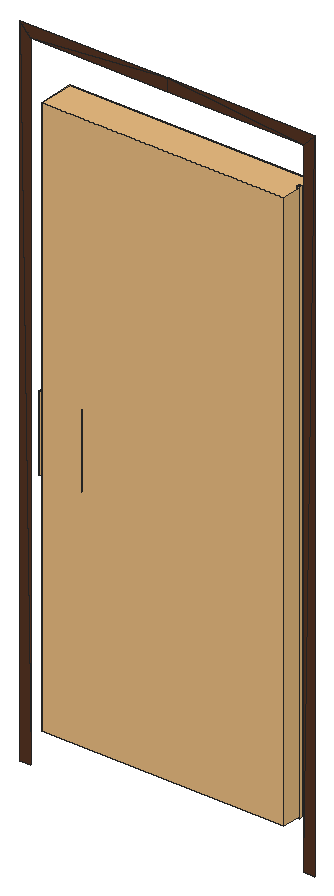
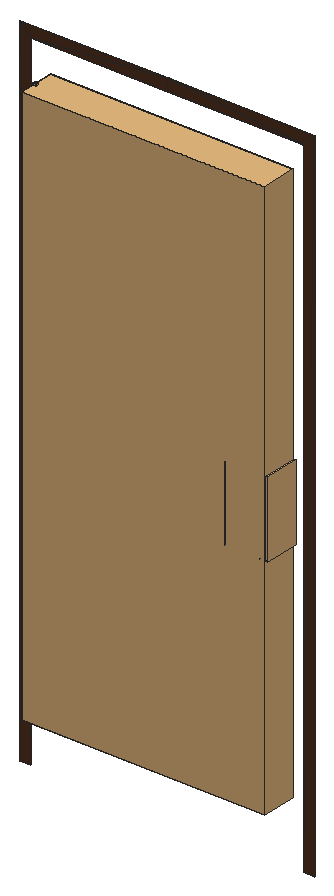
# SketchUp Ruby script. Lengths in inches.
U = 1.inch
M = Sketchup.active_model
def pt(a) = Geom::Point3d.new(a.map { |v| v * U })
def face(e, loops, mat)
  f = e.add_face(loops[0].map { |a| pt(a) })
  loops[1..].each { |l| e.add_face(l.map { |a| pt(a) }).erase! }
  f.material = f.back_material = mat if mat
  f
end
# faces: each face lists its corners as indices into pts; further lists are holes
def faces(e, pts, list, mat = nil) = list.each { |f| face(e, (f[0].is_a?(Array) ? f : [f]).map { |l| l.map { |i| pts[i] } }, mat) }
# xy, xz, yz: faces in a plane at the given z, y or x. An outline is a flat list of corners, or four numbers for a rectangle; further outlines are holes
def ring(l) = l.size == 4 ? [[l[0], l[1]], [l[2], l[1]], [l[2], l[3]], [l[0], l[3]]] : l.each_slice(2).to_a
def flat(e, list, mat, &to3) = list.each { |f| face(e, (f[0].is_a?(Array) ? f : [f]).map { |l| ring(l).map { |u, v| to3.(u, v) } }, mat) }
def xy(e, z, list, mat = nil) = flat(e, list, mat) { |x, y| [x, y, z] }
def xz(e, y, list, mat = nil) = flat(e, list, mat) { |x, z| [x, y, z] }
def yz(e, x, list, mat = nil) = flat(e, list, mat) { |y, z| [x, y, z] }
def lines(e, pts, list) = list.each { |a, b| e.add_line(pt(pts[a]), pt(pts[b])) }
# prism: a flat outline (further loops are holes) pulled along v
def prism(e, loops, v, mat = nil)
  f = face(e, loops, mat); d = Geom::Vector3d.new(v.map { |x| x * U })
  f.pushpull(f.normal.samedirection?(d) ? d.length : -d.length)
end
def box(e, o, s, mat = nil) = prism(e, [[o, [o[0] + s[0], o[1], o[2]], [o[0] + s[0], o[1] + s[1], o[2]], [o[0], o[1] + s[1], o[2]]]], [0, 0, s[2]], mat)
def at(x, y, z, deg = 0) = Geom::Transformation.translation(pt([x, y, z])) * Geom::Transformation.rotation(ORIGIN, Z_AXIS, deg.degrees)
def axes(o, x, y, z) = Geom::Transformation.new([*x, 0, *y, 0, *z, 0, *pt(o).to_a, 1])
def part(name) = M.definitions.add(name)
# library, detail: a bought-in or finely detailed component or shape, given as its bounding box
def library(name, o, s) = part(name).tap { |d| box(d.entities, o, s) }
def detail(e, o, s) = box(e.add_group.entities, o, s)
def put(e, d, t, mat = nil) = e.add_instance(d, t).tap { |i| i.material = mat if mat }
def group(e, t, mat = nil) = e.add_group.tap { |g| g.transformation = t; g.material = mat if mat }.entities
root = M.entities
M.materials.add("Material \#0").color = [86, 53, 35]
M.materials.add("Material \#1").color = [140, 140, 140]
c1 = library("3DGeom~3_Defintion",[-83.33,-500,-350],[620.1,1000,533.33])
c2 = part("3DGeom~21_Defintion")
xy(c2.entities,73.08,[[-976.3,-241.71,23.7,-241.71,-976.3,-223.46],[23.7,-241.71,5.45,-223.46,-976.3,-223.46],[23.7,-241.71,23.7,0,5.45,-223.46],[5.45,-223.46,23.7,0,5.45,0],[23.7,0,23.7,241.71,5.45,223.46],
  [5.45,0,23.7,0,5.45,223.46],[-976.3,223.46,23.7,241.71,-976.3,241.71],[-976.3,223.46,5.45,223.46,23.7,241.71]],"Material \#0")
c3 = library("3DGeom~6_Defintion",[-5.59,-471.8,-48.03],[468.87,1000,73.72])
c4 = library("3DGeom~9_Defintion",[456.52,-471.89,-18.89],[5.57,1000,5.49])
c5 = library("3DGeom~7_Defintion",[455.56,-471.94,-18.85],[5.55,1000,5.48])
c6 = part("3DGeom~8_Defintion")
xz(c6.entities,-471.94,[[458.125,-17.29,459.53,-16.11,457.73,-17.15],[458.125,-17.29,458.54,-17.29,459.53,-16.11],[458.54,-17.29,458.93,-17.15,459.53,-16.11],[457.73,-17.15,459.53,-16.11,457.42,-16.88],[458.93,-17.15,459.25,-16.88,459.53,-16.11],
  [457.42,-16.88,459.53,-16.11,457.21,-16.52],[459.25,-16.88,459.46,-16.52,459.53,-16.11],[457.21,-16.52,459.53,-16.11,457.14,-16.11],[457.14,-16.11,459.53,-16.11,457.21,-15.7],[459.53,-16.11,457.42,-15.34,457.21,-15.7],
  [459.53,-16.11,457.73,-15.07,457.42,-15.34],[459.53,-16.11,458.125,-14.93,457.73,-15.07],[459.53,-16.11,458.54,-14.93,458.125,-14.93],[459.53,-16.11,458.93,-15.07,458.54,-14.93],[459.53,-16.11,459.25,-15.34,458.93,-15.07],
  [459.53,-16.11,459.46,-15.7,459.25,-15.34]],"Material \#1")
xz(c6.entities,-416.39,[[458.125,-17.29,457.73,-17.15,459.53,-16.11],[458.125,-17.29,459.53,-16.11,458.54,-17.29],[458.54,-17.29,459.53,-16.11,458.93,-17.15],[457.73,-17.15,457.42,-16.88,459.53,-16.11],[458.93,-17.15,459.53,-16.11,459.25,-16.88],
  [457.42,-16.88,457.21,-16.52,459.53,-16.11],[459.25,-16.88,459.53,-16.11,459.46,-16.52],[457.21,-16.52,457.14,-16.11,459.53,-16.11],[457.14,-16.11,457.21,-15.7,459.53,-16.11],[459.53,-16.11,457.21,-15.7,457.42,-15.34],
  [459.53,-16.11,457.42,-15.34,457.73,-15.07],[459.53,-16.11,457.73,-15.07,458.125,-14.93],[459.53,-16.11,458.125,-14.93,458.54,-14.93],[459.53,-16.11,458.54,-14.93,458.93,-15.07],[459.53,-16.11,458.93,-15.07,459.25,-15.34],
  [459.53,-16.11,459.25,-15.34,459.46,-15.7]],"Material \#1")
xz(c6.entities,-27.5,[[458.125,-17.29,459.53,-16.11,457.73,-17.15],[458.125,-17.29,458.54,-17.29,459.53,-16.11],[458.54,-17.29,458.93,-17.15,459.53,-16.11],[457.73,-17.15,459.53,-16.11,457.42,-16.88],[458.93,-17.15,459.25,-16.88,459.53,-16.11],
  [457.42,-16.88,459.53,-16.11,457.21,-16.52],[459.25,-16.88,459.46,-16.52,459.53,-16.11],[457.21,-16.52,459.53,-16.11,457.14,-16.11],[457.14,-16.11,459.53,-16.11,457.21,-15.7],[459.53,-16.11,457.42,-15.34,457.21,-15.7],
  [459.53,-16.11,457.73,-15.07,457.42,-15.34],[459.53,-16.11,458.125,-14.93,457.73,-15.07],[459.53,-16.11,458.54,-14.93,458.125,-14.93],[459.53,-16.11,458.93,-15.07,458.54,-14.93],[459.53,-16.11,459.25,-15.34,458.93,-15.07],
  [459.53,-16.11,459.46,-15.7,459.25,-15.34]],"Material \#1")
xz(c6.entities,28.06,[[458.125,-17.29,457.73,-17.15,459.53,-16.11],[458.125,-17.29,459.53,-16.11,458.54,-17.29],[458.54,-17.29,459.53,-16.11,458.93,-17.15],[457.73,-17.15,457.42,-16.88,459.53,-16.11],[458.93,-17.15,459.53,-16.11,459.25,-16.88],
  [457.42,-16.88,457.21,-16.52,459.53,-16.11],[459.25,-16.88,459.53,-16.11,459.46,-16.52],[457.21,-16.52,457.14,-16.11,459.53,-16.11],[457.14,-16.11,457.21,-15.7,459.53,-16.11],[459.53,-16.11,457.21,-15.7,457.42,-15.34],
  [459.53,-16.11,457.42,-15.34,457.73,-15.07],[459.53,-16.11,457.73,-15.07,458.125,-14.93],[459.53,-16.11,458.125,-14.93,458.54,-14.93],[459.53,-16.11,458.54,-14.93,458.93,-15.07],[459.53,-16.11,458.93,-15.07,459.25,-15.34],
  [459.53,-16.11,459.25,-15.34,459.46,-15.7]],"Material \#1")
xz(c6.entities,472.5,[[458.125,-17.29,459.53,-16.11,457.73,-17.15],[458.125,-17.29,458.54,-17.29,459.53,-16.11],[458.54,-17.29,458.93,-17.15,459.53,-16.11],[457.73,-17.15,459.53,-16.11,457.42,-16.88],[458.93,-17.15,459.25,-16.88,459.53,-16.11],
  [457.42,-16.88,459.53,-16.11,457.21,-16.52],[459.25,-16.88,459.46,-16.52,459.53,-16.11],[457.21,-16.52,459.53,-16.11,457.14,-16.11],[457.14,-16.11,459.53,-16.11,457.21,-15.7],[459.53,-16.11,457.42,-15.34,457.21,-15.7],
  [459.53,-16.11,457.73,-15.07,457.42,-15.34],[459.53,-16.11,458.125,-14.93,457.73,-15.07],[459.53,-16.11,458.54,-14.93,458.125,-14.93],[459.53,-16.11,458.93,-15.07,458.54,-14.93],[459.53,-16.11,459.25,-15.34,458.93,-15.07],
  [459.53,-16.11,459.46,-15.7,459.25,-15.34]],"Material \#1")
xz(c6.entities,528.06,[[458.125,-17.29,457.73,-17.15,459.53,-16.11],[458.125,-17.29,459.53,-16.11,458.54,-17.29],[458.54,-17.29,459.53,-16.11,458.93,-17.15],[457.73,-17.15,457.42,-16.88,459.53,-16.11],[458.93,-17.15,459.53,-16.11,459.25,-16.88],
  [457.42,-16.88,457.21,-16.52,459.53,-16.11],[459.25,-16.88,459.53,-16.11,459.46,-16.52],[457.21,-16.52,457.14,-16.11,459.53,-16.11],[457.14,-16.11,457.21,-15.7,459.53,-16.11],[459.53,-16.11,457.21,-15.7,457.42,-15.34],
  [459.53,-16.11,457.42,-15.34,457.73,-15.07],[459.53,-16.11,457.73,-15.07,458.125,-14.93],[459.53,-16.11,458.125,-14.93,458.54,-14.93],[459.53,-16.11,458.54,-14.93,458.93,-15.07],[459.53,-16.11,458.93,-15.07,459.25,-15.34],
  [459.53,-16.11,459.25,-15.34,459.46,-15.7]],"Material \#1")
xy(root,9.094,[[138.948,197.844,138.952,197.861,138.889,197.864],[138.948,197.844,139.008,197.861,138.952,197.861],[138.948,197.844,139.011,197.844,139.008,197.861],[139.011,197.844,139.061,197.878,139.008,197.861],[139.011,197.844,139.07,197.864,139.061,197.878],
  [138.952,197.861,138.898,197.878,138.889,197.864],[138.889,197.864,138.898,197.878,138.841,197.901],[139.07,197.864,139.104,197.912,139.061,197.878],[139.07,197.864,139.118,197.901,139.104,197.912],[138.898,197.878,138.855,197.912,138.841,197.901],
  [138.841,197.901,138.855,197.912,138.81,197.952],[139.118,197.901,139.132,197.958,139.104,197.912],[139.118,197.901,139.149,197.952,139.132,197.958],[138.855,197.912,138.827,197.958,138.81,197.952],[138.81,197.952,138.827,197.958,138.799,198.009],
  [139.149,197.952,139.142,198.009,139.132,197.958],[139.149,197.952,139.16,198.009,139.142,198.009],[138.827,197.958,138.817,198.009,138.799,198.009],[138.799,198.009,138.817,198.009,138.81,198.067],[138.817,198.009,138.827,198.061,138.81,198.067],
  [139.142,198.009,139.16,198.009,139.132,198.061],[139.16,198.009,139.149,198.067,139.132,198.061],[138.827,198.061,138.841,198.117,138.81,198.067],[138.827,198.061,138.855,198.106,138.841,198.117],[139.132,198.061,139.149,198.067,139.104,198.106],
  [139.149,198.067,139.118,198.117,139.104,198.106],[138.855,198.106,138.889,198.155,138.841,198.117],[138.855,198.106,138.898,198.14,138.889,198.155],[139.104,198.106,139.118,198.117,139.061,198.14],[139.118,198.117,139.07,198.155,139.061,198.14],
  [138.898,198.14,138.948,198.175,138.889,198.155],[138.898,198.14,138.952,198.158,138.948,198.175],[139.061,198.14,139.07,198.155,139.008,198.158],[139.07,198.155,139.011,198.175,139.008,198.158],[138.952,198.158,139.011,198.175,138.948,198.175],
  [138.952,198.158,139.008,198.158,139.011,198.175]],"Material \#1")
xy(root,9.11,[[138.948,197.844,138.889,197.864,138.898,197.878],[138.948,197.844,138.898,197.878,138.952,197.861],[138.948,197.844,138.952,197.861,139.011,197.844],[139.011,197.844,138.952,197.861,139.008,197.861],[139.011,197.844,139.008,197.861,139.07,197.864],
  [139.008,197.861,139.061,197.878,139.07,197.864],[138.889,197.864,138.841,197.901,138.855,197.912],[138.889,197.864,138.855,197.912,138.898,197.878],[139.07,197.864,139.061,197.878,139.118,197.901],[139.061,197.878,139.104,197.912,139.118,197.901],
  [138.841,197.901,138.81,197.952,138.827,197.958],[138.841,197.901,138.827,197.958,138.855,197.912],[139.118,197.901,139.104,197.912,139.149,197.952],[139.104,197.912,139.132,197.958,139.149,197.952],[138.81,197.952,138.799,198.009,138.817,198.009],
  [138.81,197.952,138.817,198.009,138.827,197.958],[139.149,197.952,139.132,197.958,139.16,198.009],[139.132,197.958,139.142,198.009,139.16,198.009],[138.799,198.009,138.81,198.067,138.827,198.061],[138.799,198.009,138.827,198.061,138.817,198.009],
  [139.142,198.009,139.132,198.061,139.149,198.067],[139.142,198.009,139.149,198.067,139.16,198.009],[138.827,198.061,138.81,198.067,138.855,198.106],[139.132,198.061,139.104,198.106,139.118,198.117],[139.132,198.061,139.118,198.117,139.149,198.067],
  [138.81,198.067,138.841,198.117,138.855,198.106],[138.855,198.106,138.841,198.117,138.898,198.14],[139.104,198.106,139.061,198.14,139.07,198.155],[139.104,198.106,139.07,198.155,139.118,198.117],[138.841,198.117,138.889,198.155,138.898,198.14],
  [138.898,198.14,138.889,198.155,138.952,198.158],[139.061,198.14,139.008,198.158,139.011,198.175],[139.061,198.14,139.011,198.175,139.07,198.155],[138.889,198.155,138.948,198.175,138.952,198.158],[138.952,198.158,138.948,198.175,139.008,198.158],
  [139.008,198.158,138.948,198.175,139.011,198.175]],"Material \#1")
xy(root,12.631,[[138.948,197.844,138.898,197.878,138.889,197.864],[138.948,197.844,138.952,197.861,138.898,197.878],[138.948,197.844,139.011,197.844,138.952,197.861],[139.011,197.844,139.008,197.861,138.952,197.861],[139.011,197.844,139.07,197.864,139.008,197.861],
  [139.008,197.861,139.07,197.864,139.061,197.878],[138.889,197.864,138.855,197.912,138.841,197.901],[138.889,197.864,138.898,197.878,138.855,197.912],[139.07,197.864,139.118,197.901,139.061,197.878],[139.061,197.878,139.118,197.901,139.104,197.912],
  [138.841,197.901,138.827,197.958,138.81,197.952],[138.841,197.901,138.855,197.912,138.827,197.958],[139.118,197.901,139.149,197.952,139.104,197.912],[139.104,197.912,139.149,197.952,139.132,197.958],[138.81,197.952,138.817,198.009,138.799,198.009],
  [138.81,197.952,138.827,197.958,138.817,198.009],[139.149,197.952,139.16,198.009,139.132,197.958],[139.132,197.958,139.16,198.009,139.142,198.009],[138.799,198.009,138.817,198.009,138.827,198.061],[138.799,198.009,138.827,198.061,138.81,198.067],
  [139.142,198.009,139.149,198.067,139.132,198.061],[139.142,198.009,139.16,198.009,139.149,198.067],[138.827,198.061,138.855,198.106,138.81,198.067],[139.132,198.061,139.118,198.117,139.104,198.106],[139.132,198.061,139.149,198.067,139.118,198.117],
  [138.81,198.067,138.855,198.106,138.841,198.117],[138.855,198.106,138.898,198.14,138.841,198.117],[139.104,198.106,139.07,198.155,139.061,198.14],[139.104,198.106,139.118,198.117,139.07,198.155],[138.841,198.117,138.898,198.14,138.889,198.155],
  [138.898,198.14,138.952,198.158,138.889,198.155],[139.061,198.14,139.011,198.175,139.008,198.158],[139.061,198.14,139.07,198.155,139.011,198.175],[138.889,198.155,138.952,198.158,138.948,198.175],[138.952,198.158,139.008,198.158,138.948,198.175],
  [139.008,198.158,139.011,198.175,138.948,198.175]],"Material \#1")
xy(root,12.646,[[138.948,197.844,138.889,197.864,138.952,197.861],[138.948,197.844,138.952,197.861,139.008,197.861],[138.948,197.844,139.008,197.861,139.011,197.844],[139.011,197.844,139.008,197.861,139.061,197.878],[139.011,197.844,139.061,197.878,139.07,197.864],
  [138.952,197.861,138.889,197.864,138.898,197.878],[138.889,197.864,138.841,197.901,138.898,197.878],[139.07,197.864,139.061,197.878,139.104,197.912],[139.07,197.864,139.104,197.912,139.118,197.901],[138.898,197.878,138.841,197.901,138.855,197.912],
  [138.841,197.901,138.81,197.952,138.855,197.912],[139.118,197.901,139.104,197.912,139.132,197.958],[139.118,197.901,139.132,197.958,139.149,197.952],[138.855,197.912,138.81,197.952,138.827,197.958],[138.81,197.952,138.799,198.009,138.827,197.958],
  [139.149,197.952,139.132,197.958,139.142,198.009],[139.149,197.952,139.142,198.009,139.16,198.009],[138.827,197.958,138.799,198.009,138.817,198.009],[138.799,198.009,138.81,198.067,138.817,198.009],[138.817,198.009,138.81,198.067,138.827,198.061],
  [139.142,198.009,139.132,198.061,139.16,198.009],[139.16,198.009,139.132,198.061,139.149,198.067],[138.827,198.061,138.81,198.067,138.841,198.117],[138.827,198.061,138.841,198.117,138.855,198.106],[139.132,198.061,139.104,198.106,139.149,198.067],
  [139.149,198.067,139.104,198.106,139.118,198.117],[138.855,198.106,138.841,198.117,138.889,198.155],[138.855,198.106,138.889,198.155,138.898,198.14],[139.104,198.106,139.061,198.14,139.118,198.117],[139.118,198.117,139.061,198.14,139.07,198.155],
  [138.898,198.14,138.889,198.155,138.948,198.175],[138.898,198.14,138.948,198.175,138.952,198.158],[139.061,198.14,139.008,198.158,139.07,198.155],[139.07,198.155,139.008,198.158,139.011,198.175],[138.952,198.158,138.948,198.175,139.011,198.175],
  [138.952,198.158,139.011,198.175,139.008,198.158]],"Material \#1")
xy(root,40.496,[[138.948,197.844,138.952,197.861,138.889,197.864],[138.948,197.844,139.008,197.861,138.952,197.861],[138.948,197.844,139.011,197.844,139.008,197.861],[139.011,197.844,139.061,197.878,139.008,197.861],[139.011,197.844,139.07,197.864,139.061,197.878],
  [138.952,197.861,138.898,197.878,138.889,197.864],[138.889,197.864,138.898,197.878,138.841,197.901],[139.07,197.864,139.104,197.912,139.061,197.878],[139.07,197.864,139.118,197.901,139.104,197.912],[138.898,197.878,138.855,197.912,138.841,197.901],
  [138.841,197.901,138.855,197.912,138.81,197.952],[139.118,197.901,139.132,197.958,139.104,197.912],[139.118,197.901,139.149,197.952,139.132,197.958],[138.855,197.912,138.827,197.958,138.81,197.952],[138.81,197.952,138.827,197.958,138.799,198.009],
  [139.149,197.952,139.142,198.009,139.132,197.958],[139.149,197.952,139.16,198.009,139.142,198.009],[138.827,197.958,138.817,198.009,138.799,198.009],[138.799,198.009,138.817,198.009,138.81,198.067],[138.817,198.009,138.827,198.061,138.81,198.067],
  [139.142,198.009,139.16,198.009,139.132,198.061],[139.16,198.009,139.149,198.067,139.132,198.061],[138.827,198.061,138.841,198.117,138.81,198.067],[138.827,198.061,138.855,198.106,138.841,198.117],[139.132,198.061,139.149,198.067,139.104,198.106],
  [139.149,198.067,139.118,198.117,139.104,198.106],[138.855,198.106,138.889,198.155,138.841,198.117],[138.855,198.106,138.898,198.14,138.889,198.155],[139.104,198.106,139.118,198.117,139.061,198.14],[139.118,198.117,139.07,198.155,139.061,198.14],
  [138.898,198.14,138.948,198.175,138.889,198.155],[138.898,198.14,138.952,198.158,138.948,198.175],[139.061,198.14,139.07,198.155,139.008,198.158],[139.07,198.155,139.011,198.175,139.008,198.158],[138.952,198.158,139.011,198.175,138.948,198.175],
  [138.952,198.158,139.008,198.158,139.011,198.175]],"Material \#1")
xy(root,40.511,[[138.948,197.844,138.889,197.864,138.898,197.878],[138.948,197.844,138.898,197.878,138.952,197.861],[138.948,197.844,138.952,197.861,139.011,197.844],[139.011,197.844,138.952,197.861,139.008,197.861],[139.011,197.844,139.008,197.861,139.07,197.864],
  [139.008,197.861,139.061,197.878,139.07,197.864],[138.889,197.864,138.841,197.901,138.855,197.912],[138.889,197.864,138.855,197.912,138.898,197.878],[139.07,197.864,139.061,197.878,139.118,197.901],[139.061,197.878,139.104,197.912,139.118,197.901],
  [138.841,197.901,138.81,197.952,138.827,197.958],[138.841,197.901,138.827,197.958,138.855,197.912],[139.118,197.901,139.104,197.912,139.149,197.952],[139.104,197.912,139.132,197.958,139.149,197.952],[138.81,197.952,138.799,198.009,138.817,198.009],
  [138.81,197.952,138.817,198.009,138.827,197.958],[139.149,197.952,139.132,197.958,139.16,198.009],[139.132,197.958,139.142,198.009,139.16,198.009],[138.799,198.009,138.81,198.067,138.827,198.061],[138.799,198.009,138.827,198.061,138.817,198.009],
  [139.142,198.009,139.132,198.061,139.149,198.067],[139.142,198.009,139.149,198.067,139.16,198.009],[138.827,198.061,138.81,198.067,138.855,198.106],[139.132,198.061,139.104,198.106,139.118,198.117],[139.132,198.061,139.118,198.117,139.149,198.067],
  [138.81,198.067,138.841,198.117,138.855,198.106],[138.855,198.106,138.841,198.117,138.898,198.14],[139.104,198.106,139.061,198.14,139.07,198.155],[139.104,198.106,139.07,198.155,139.118,198.117],[138.841,198.117,138.889,198.155,138.898,198.14],
  [138.898,198.14,138.889,198.155,138.952,198.158],[139.061,198.14,139.008,198.158,139.011,198.175],[139.061,198.14,139.011,198.175,139.07,198.155],[138.889,198.155,138.948,198.175,138.952,198.158],[138.952,198.158,138.948,198.175,139.008,198.158],
  [139.008,198.158,138.948,198.175,139.011,198.175]],"Material \#1")
xy(root,44.032,[[138.948,197.844,138.898,197.878,138.889,197.864],[138.948,197.844,138.952,197.861,138.898,197.878],[138.948,197.844,139.011,197.844,138.952,197.861],[139.011,197.844,139.008,197.861,138.952,197.861],[139.011,197.844,139.07,197.864,139.008,197.861],
  [139.008,197.861,139.07,197.864,139.061,197.878],[138.889,197.864,138.855,197.912,138.841,197.901],[138.889,197.864,138.898,197.878,138.855,197.912],[139.07,197.864,139.118,197.901,139.061,197.878],[139.061,197.878,139.118,197.901,139.104,197.912],
  [138.841,197.901,138.827,197.958,138.81,197.952],[138.841,197.901,138.855,197.912,138.827,197.958],[139.118,197.901,139.149,197.952,139.104,197.912],[139.104,197.912,139.149,197.952,139.132,197.958],[138.81,197.952,138.817,198.009,138.799,198.009],
  [138.81,197.952,138.827,197.958,138.817,198.009],[139.149,197.952,139.16,198.009,139.132,197.958],[139.132,197.958,139.16,198.009,139.142,198.009],[138.799,198.009,138.817,198.009,138.827,198.061],[138.799,198.009,138.827,198.061,138.81,198.067],
  [139.142,198.009,139.149,198.067,139.132,198.061],[139.142,198.009,139.16,198.009,139.149,198.067],[138.827,198.061,138.855,198.106,138.81,198.067],[139.132,198.061,139.118,198.117,139.104,198.106],[139.132,198.061,139.149,198.067,139.118,198.117],
  [138.81,198.067,138.855,198.106,138.841,198.117],[138.855,198.106,138.898,198.14,138.841,198.117],[139.104,198.106,139.07,198.155,139.061,198.14],[139.104,198.106,139.118,198.117,139.07,198.155],[138.841,198.117,138.898,198.14,138.889,198.155],
  [138.898,198.14,138.952,198.158,138.889,198.155],[139.061,198.14,139.011,198.175,139.008,198.158],[139.061,198.14,139.07,198.155,139.011,198.175],[138.889,198.155,138.952,198.158,138.948,198.175],[138.952,198.158,139.008,198.158,138.948,198.175],
  [139.008,198.158,139.011,198.175,138.948,198.175]],"Material \#1")
xy(root,44.048,[[138.948,197.844,138.889,197.864,138.952,197.861],[138.948,197.844,138.952,197.861,139.008,197.861],[138.948,197.844,139.008,197.861,139.011,197.844],[139.011,197.844,139.008,197.861,139.061,197.878],[139.011,197.844,139.061,197.878,139.07,197.864],
  [138.952,197.861,138.889,197.864,138.898,197.878],[138.889,197.864,138.841,197.901,138.898,197.878],[139.07,197.864,139.061,197.878,139.104,197.912],[139.07,197.864,139.104,197.912,139.118,197.901],[138.898,197.878,138.841,197.901,138.855,197.912],
  [138.841,197.901,138.81,197.952,138.855,197.912],[139.118,197.901,139.104,197.912,139.132,197.958],[139.118,197.901,139.132,197.958,139.149,197.952],[138.855,197.912,138.81,197.952,138.827,197.958],[138.81,197.952,138.799,198.009,138.827,197.958],
  [139.149,197.952,139.132,197.958,139.142,198.009],[139.149,197.952,139.142,198.009,139.16,198.009],[138.827,197.958,138.799,198.009,138.817,198.009],[138.799,198.009,138.81,198.067,138.817,198.009],[138.817,198.009,138.81,198.067,138.827,198.061],
  [139.142,198.009,139.132,198.061,139.16,198.009],[139.16,198.009,139.132,198.061,139.149,198.067],[138.827,198.061,138.81,198.067,138.841,198.117],[138.827,198.061,138.841,198.117,138.855,198.106],[139.132,198.061,139.104,198.106,139.149,198.067],
  [139.149,198.067,139.104,198.106,139.118,198.117],[138.855,198.106,138.841,198.117,138.889,198.155],[138.855,198.106,138.889,198.155,138.898,198.14],[139.104,198.106,139.061,198.14,139.118,198.117],[139.118,198.117,139.061,198.14,139.07,198.155],
  [138.898,198.14,138.889,198.155,138.948,198.175],[138.898,198.14,138.948,198.175,138.952,198.158],[139.061,198.14,139.008,198.158,139.07,198.155],[139.07,198.155,139.008,198.158,139.011,198.175],[138.952,198.158,138.948,198.175,139.011,198.175],
  [138.952,198.158,139.011,198.175,139.008,198.158]],"Material \#1")
xz(root,197.036,[[109.325,40.152,109.188,40.447,109.238,40.453],[109.238,40.453,109.283,40.471,109.331,40.461],[109.384,40.524,109.415,40.581,109.401,40.551],[109.384,40.524,109.431,40.647,109.415,40.581],[109.383,40.579,109.399,40.628,109.431,40.647],
  [109.415,40.581,109.431,40.647,109.425,40.613],[109.399,40.628,109.405,40.682,109.431,40.647],[109.431,40.647,109.38,40.849,109.427,40.743],[109.431,40.647,109.399,40.736,109.38,40.849],[109.431,40.647,109.405,40.682,109.399,40.736],
  [109.431,40.647,109.427,40.743,109.434,40.682],[109.399,40.736,109.383,40.786,109.38,40.849],[109.427,40.743,109.38,40.849,109.409,40.8],[109.383,40.786,109.357,40.829,109.38,40.849],[109.357,40.829,109.324,40.866,109.38,40.849],
  [109.38,40.849,109.188,40.949,109.296,40.922],[109.38,40.849,109.283,40.894,109.188,40.949],[109.38,40.849,109.324,40.866,109.283,40.894],[109.38,40.849,109.296,40.922,109.342,40.89],[109.283,40.894,109.238,40.912,109.188,40.949],
  [109.238,40.912,109.188,40.918,109.188,40.949],[109.296,40.922,109.188,40.949,109.244,40.942]],"Material \#1")
xz(root,198.379,[[109.188,40.003,109.22,40.007,109.248,40.018],[109.128,40.018,109.248,40.018,109.322,40.118],[109.248,40.018,109.274,40.036,109.295,40.059],[109.248,40.018,109.295,40.059,109.322,40.118],[109.295,40.059,109.311,40.087,109.322,40.118],
  [109.322,40.118,109.325,40.152,109.046,40.46],[109.325,40.152,109.188,40.447,109.138,40.453],[109.325,40.152,109.238,40.453,109.188,40.447],[109.325,40.152,109.325,40.4375,109.238,40.453],[109.325,40.4375,109.327,40.45,109.238,40.453],
  [109.325,40.4375,109.326,40.444,109.327,40.45],[109.327,40.45,109.331,40.461,109.238,40.453],[109.327,40.45,109.328,40.456,109.331,40.461],[109.238,40.453,109.331,40.461,109.283,40.471],[109.331,40.461,109.324,40.498,109.283,40.471],
  [109.331,40.461,109.357,40.535,109.324,40.498],[109.331,40.461,109.334,40.466,109.431,40.647],[109.331,40.461,109.431,40.647,109.357,40.535],[109.334,40.466,109.338,40.47,109.431,40.647],[109.338,40.47,109.342,40.475,109.384,40.524],
  [109.338,40.47,109.384,40.524,109.431,40.647],[109.342,40.475,109.364,40.498,109.384,40.524],[109.384,40.524,109.401,40.551,109.415,40.581],[109.384,40.524,109.415,40.581,109.431,40.647],[109.357,40.535,109.431,40.647,109.383,40.579],
  [109.383,40.579,109.431,40.647,109.399,40.628],[109.415,40.581,109.425,40.613,109.431,40.647],[109.399,40.628,109.431,40.647,109.405,40.682],[109.431,40.647,109.38,40.849,109.399,40.736],[109.431,40.647,109.427,40.743,109.38,40.849],
  [109.431,40.647,109.399,40.736,109.405,40.682],[109.431,40.647,109.434,40.682,109.427,40.743],[109.399,40.736,109.38,40.849,109.383,40.786],[109.427,40.743,109.409,40.8,109.38,40.849],[109.383,40.786,109.38,40.849,109.357,40.829],
  [109.357,40.829,109.38,40.849,109.324,40.866],[109.38,40.849,109.188,40.949,109.283,40.894],[109.38,40.849,109.296,40.922,109.188,40.949],[109.38,40.849,109.283,40.894,109.324,40.866],[109.38,40.849,109.342,40.89,109.296,40.922],
  [109.283,40.894,109.188,40.949,109.238,40.912],[109.238,40.912,109.188,40.949,109.188,40.918],[109.296,40.922,109.244,40.942,109.188,40.949]],"Material \#1")
xz(root,198.681,[[109.302,37.652,109.3,37.663,109.405,37.695],[109.302,37.652,109.405,37.695,109.408,37.684],[109.408,37.684,109.405,37.695,109.501,37.745],[109.408,37.684,109.501,37.745,109.507,37.734],[109.507,37.734,109.501,37.745,109.588,37.811],
  [109.507,37.734,109.588,37.811,109.595,37.802],[109.226,37.828,109.224,37.84,109.257,37.85],[109.226,37.828,109.257,37.85,109.261,37.839],[109.261,37.839,109.257,37.85,109.288,37.866],[109.261,37.839,109.288,37.866,109.294,37.855],
  [109.671,37.885,109.663,37.893,109.724,37.987],[109.671,37.885,109.724,37.987,109.733,37.981],[109.733,37.981,109.724,37.987,109.77,38.092],[109.733,37.981,109.77,38.092,109.78,38.088],[109.78,38.088,109.77,38.092,109.799,38.206],
  [109.78,38.088,109.799,38.206,109.809,38.204]],"Material \#1")
yz(root,109.209,[[198.412,40.612,198.412,40.639,198.724,40.612],[198.724,40.612,198.412,40.639,198.724,40.639]],"Material \#1")
yz(root,109.214,[[198.412,40.721,198.412,40.773,198.724,40.721]],"Material \#1")
yz(root,109.217,[[198.412,40.661,198.412,40.684,198.724,40.661],[198.724,40.661,198.412,40.684,198.724,40.684]],"Material \#1")
p = [[109.199,198.412,40.549],[109.202,198.724,40.553],[109.209,198.724,40.525],[109.209,198.724,40.525],[109.209,198.412,40.525],[109.199,198.412,40.549],
  [109.209,198.412,40.612],[109.209,198.724,40.612],[109.202,198.724,40.578],[109.209,198.724,40.639],[109.209,198.412,40.639],[109.217,198.412,40.661],
  [109.217,198.412,40.661],[109.217,198.724,40.661],[109.209,198.724,40.639],[109.209,198.724,40.706],[109.209,198.412,40.706],[109.214,198.412,40.721],
  [109.209,198.412,40.706],[109.209,198.724,40.706],[109.217,198.724,40.684],[109.214,198.412,40.721],[109.214,198.724,40.721],[109.209,198.724,40.706],
  [109.214,198.412,40.773],[109.212,198.724,40.782],[109.214,198.724,40.721],[109.217,198.724,40.684],[109.217,198.412,40.684],[109.209,198.412,40.706],
  [109.212,198.724,40.782],[109.214,198.412,40.788],[109.214,198.412,40.839],[109.214,198.412,40.839],[109.214,198.724,40.839],[109.212,198.724,40.782]]
faces(root,p,[[0,1,2],[3,4,5],[6,7,8],[9,10,11],[12,13,14],[15,16,17],[18,19,20],[21,22,23],
  [24,25,26],[27,28,29],[30,31,32],[33,34,35]],"Material \#1")
put(root,c1,axes([109.1875,197.04,42.25],[0.00867,0,0],[0,0,0.00942],[0,-0.00806,0]),"Material \#1")
put(root,c2,axes([122.55,192.81,83.86],[0,0,0.08282],[0.07619,0,0],[0,0.07084,0]),"Material \#0")
put(root,c3,axes([109.1875,197.04,42.25],[0.06466,0,0],[0,0,0.07028],[0,-0.06011,0]),"Material \#1")
put(root,c4,axes([109.1875,197.04,42.25],[0.06486,0,0],[0,0,0.07051],[0,-0.0603,0]),"Material \#1")
put(root,c5,axes([109.1875,197.04,42.25],[0.065,0,0],[0,0,0.07065],[0,-0.06043,0]),"Material \#1")
put(root,c6,axes([109.1875,197.04,42.25],[0.065,0,0],[0,0,0.07065],[0,-0.06043,0]),"Material \#1")
